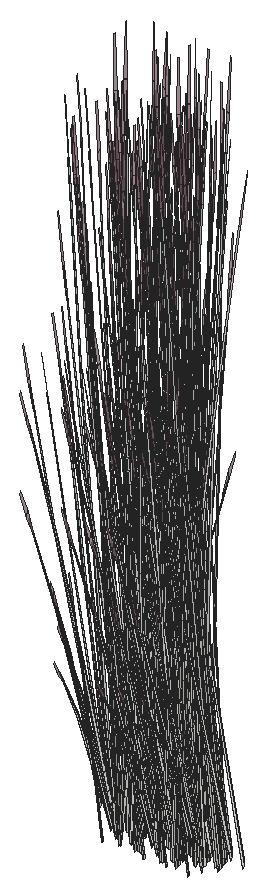
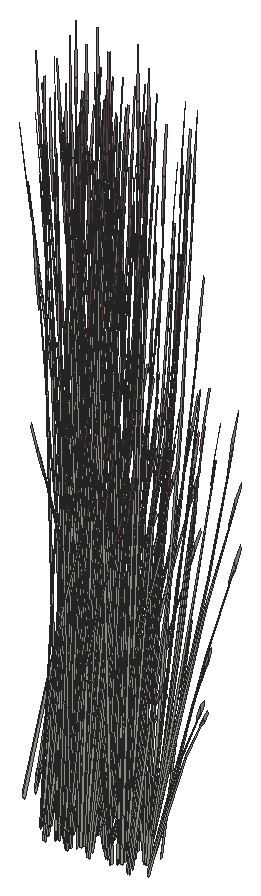
# SketchUp Ruby script. Lengths in inches.
U = 1.inch
M = Sketchup.active_model
def pt(a) = Geom::Point3d.new(a.map { |v| v * U })
def face(e, loops, mat)
  f = e.add_face(loops[0].map { |a| pt(a) })
  loops[1..].each { |l| e.add_face(l.map { |a| pt(a) }).erase! }
  f.material = f.back_material = mat if mat
  f
end
# faces: each face lists its corners as indices into pts; further lists are holes
def faces(e, pts, list, mat = nil) = list.each { |f| face(e, (f[0].is_a?(Array) ? f : [f]).map { |l| l.map { |i| pts[i] } }, mat) }
# xy, xz, yz: faces in a plane at the given z, y or x. An outline is a flat list of corners, or four numbers for a rectangle; further outlines are holes
def ring(l) = l.size == 4 ? [[l[0], l[1]], [l[2], l[1]], [l[2], l[3]], [l[0], l[3]]] : l.each_slice(2).to_a
def flat(e, list, mat, &to3) = list.each { |f| face(e, (f[0].is_a?(Array) ? f : [f]).map { |l| ring(l).map { |u, v| to3.(u, v) } }, mat) }
def xy(e, z, list, mat = nil) = flat(e, list, mat) { |x, y| [x, y, z] }
def xz(e, y, list, mat = nil) = flat(e, list, mat) { |x, z| [x, y, z] }
def yz(e, x, list, mat = nil) = flat(e, list, mat) { |y, z| [x, y, z] }
def lines(e, pts, list) = list.each { |a, b| e.add_line(pt(pts[a]), pt(pts[b])) }
# prism: a flat outline (further loops are holes) pulled along v
def prism(e, loops, v, mat = nil)
  f = face(e, loops, mat); d = Geom::Vector3d.new(v.map { |x| x * U })
  f.pushpull(f.normal.samedirection?(d) ? d.length : -d.length)
end
def box(e, o, s, mat = nil) = prism(e, [[o, [o[0] + s[0], o[1], o[2]], [o[0] + s[0], o[1] + s[1], o[2]], [o[0], o[1] + s[1], o[2]]]], [0, 0, s[2]], mat)
def at(x, y, z, deg = 0) = Geom::Transformation.translation(pt([x, y, z])) * Geom::Transformation.rotation(ORIGIN, Z_AXIS, deg.degrees)
def axes(o, x, y, z) = Geom::Transformation.new([*x, 0, *y, 0, *z, 0, *pt(o).to_a, 1])
def part(name) = M.definitions.add(name)
# library, detail: a bought-in or finely detailed component or shape, given as its bounding box
def library(name, o, s) = part(name).tap { |d| box(d.entities, o, s) }
def detail(e, o, s) = box(e.add_group.entities, o, s)
def put(e, d, t, mat = nil) = e.add_instance(d, t).tap { |i| i.material = mat if mat }
def group(e, t, mat = nil) = e.add_group.tap { |g| g.transformation = t; g.material = mat if mat }.entities
root = M.entities
M.materials.add("LightPink_Translucent").color = [144, 107, 117]
M.materials["LightPink_Translucent"].alpha = 0.75
c1 = part("blade")
p = [[2.15,0.21,22],[0,0.17,0],[0.09,0.45,0],[2.18,0.31,22],[2.29,0.31,22],[0.38,0.45,0],
  [2.48,0.24,33],[2.49,0.24,33],[2.48,0.22,33]]
faces(c1.entities,p,[[0,1,2,3],[4,5,2,3],[6,3,4,7],[8,0,3,6]])
c2 = part("seeds")
p = [[0.3,-0.1,1.38],[-0.01,-0.03,1.59],[-0.01,-0.03,0.03],[0.14,-0.07,-0.07],[0.29,-0.03,3],[0.15,0.01,3.11]]
faces(c2.entities,p,[[0,1,2,3],[1,0,4,5]],"LightPink_Translucent")
c3 = part("blade with seeds")
put(c3.entities,c1,at(0,0,0))
put(c3.entities,c2,axes([2.4,0.25,30.99],[1.5799,-0.05474,1.17369],[-0.12525,1.92788,0.29478],[-0.07173,-0.02425,1.56792]))
put(root,c3,axes([336.72,354.52,621.875],[0.14639,-0.01056,1.71376],[-0.09712,0.45778,0.13857],[-0.20862,-0.02831,0.73262]))
put(root,c3,axes([337.16,354.09,622.98],[-0.35281,-0.01123,-0.71045],[0.0237,-0.47284,0.08574],[-0.14947,-0.0499,1.00501]))
put(root,c3,axes([336.875,354.21,620.59],[0.06891,0.12984,1.43002],[-0.15879,0.35293,-0.30754],[-0.16304,-0.08436,0.61141]))
put(root,c3,axes([336.59,354.91,622.53],[-0.29332,-0.1301,-0.35414],[0.08555,-0.37955,0.4572],[-0.11809,0.0348,0.87481]))
put(root,c3,axes([337.04,354.1875,622.68],[-0.25628,0.30892,-0.51099],[-0.22444,-0.32634,-0.3958],[-0.13021,-0.047,0.97773]))
put(root,c3,axes([336.63,355.08,619.49],[0.00895,0.0735,1.76342],[-0.18044,0.38382,-0.26939],[-0.12817,-0.01935,0.30037]))
put(root,c3,axes([336.68,353.32,622.71],[0.02617,0.04654,1.77383],[-0.12614,0.41836,-0.16761],[-0.12775,0.00303,0.31391]))
put(root,c3,axes([336.66,354.86,622.73],[0.09971,-0.42522,0.48003],[0.32782,0.1454,0.3958],[-0.12892,0.02555,0.9933]))
put(root,c3,axes([337.18,353.87,623.03],[-0.0189,0.47427,-0.1216],[-0.35781,-0.01296,-0.67495],[-0.13781,-0.03295,1.02557]))
put(root,c3,axes([336.64,354.75,622.73],[-0.12963,-0.31798,0.0643],[0.23638,-0.15564,0.50621],[-0.1042,0.03071,0.77189]))
put(root,c3,axes([336.46,354.6,620.77],[0.22533,-0.03337,1.1486],[-0.14293,0.29403,0.84392],[-0.11135,-0.04411,0.25299]))
put(root,c3,axes([336.9,354.87,623.05],[0.29332,0.1301,0.35414],[-0.08555,0.37955,-0.4572],[-0.11809,0.0348,0.87481]))
put(root,c3,axes([337.81,355.75,620.06],[-0.36714,-0.07646,-0.62353],[0.07747,-0.47163,-0.16365],[-0.10956,-0.05715,1.37633]))
put(root,c3,axes([337.23,354.05,623.05],[0.20082,0.29199,0.35414],[-0.2293,0.2764,-0.4572],[-0.1165,-0.04206,0.87481]))
put(root,c3,axes([337.33,356.64,620.02],[-0.33032,-0.23318,-0.49651],[0.19744,-0.41812,0],[-0.07523,-0.05311,1.57504]))
put(root,c3,axes([336.97,353.4,620.13],[-0.10181,0.3808,-0.03893],[-0.31336,-0.11714,-0.17649],[-0.04758,-0.06228,0.58215]))
put(root,c3,axes([338.23,355.82,620.67],[-0.35635,0.30962,-0.29095],[-0.23697,-0.43749,-0.50002],[-0.08792,-0.04443,1.59708]))
put(root,c3,axes([336.8,355.14,620.375],[-0.44133,0,0],[0,-0.52122,-0.51607],[0,-0.11871,1.63711]))
put(root,c3,axes([337.42,356.46,620.03],[-0.08291,-0.40636,-0.30978],[0.32928,-0.11539,0.30978],[-0.06638,-0.04686,1.38974]))
put(root,c3,axes([337.14,355,620.33],[-0.32829,0.39208,0.30756],[-0.32849,-0.38796,-0.36492],[-0.01146,-0.11134,1.64885]))
put(root,c3,axes([338,355.6,620.21],[-0.21202,-0.39143,-0.44739],[0.32115,-0.27564,0.21531],[-0.06861,-0.04843,1.43643]))
put(root,c3,axes([340.4,354.44,621.875],[0.14639,-0.01056,1.71376],[-0.09712,0.45778,0.13857],[-0.20862,-0.02831,0.73262]))
put(root,c3,axes([338.03,355.82,620.4375],[0.09355,-0.55261,-0.23429],[0.44354,0.09633,0.51271],[-0.0775,-0.07631,1.5644]))
put(root,c3,axes([338.19,355.95,620.62],[-0.06809,0.4162,0.1448],[-0.33266,-0.07225,-0.41347],[-0.06054,-0.04274,1.26744]))
put(root,c3,axes([337.07,355.22,620.48],[0,0.46636,0.49651],[-0.39487,0,0],[0,-0.10622,1.57504]))
put(root,c3,axes([337.93,355.33,620.67],[-0.39748,-0.22252,-0.29095],[0.19139,-0.46966,-0.50002],[-0.01249,-0.11531,1.59708]))
put(root,c3,axes([341.16,354.77,621.34],[0.10032,-0.06746,1.77064],[0.0346,0.47103,0.13857],[-0.2173,0.0625,0.63284]))
put(root,c3,axes([337.07,354.8,620.03],[0.24637,-0.29097,-0.30978],[0.24637,0.29097,0.30978],[0,-0.09372,1.38974]))
put(root,c3,axes([338.08,355.55,620.36],[0.44609,0.09826,0.45755],[-0.09078,0.55493,0.17955],[-0.06519,-0.05359,1.58856]))
put(root,c3,axes([340.84,354.02,622.98],[-0.35281,-0.01123,-0.71045],[0.0237,-0.47284,0.08574],[-0.14947,-0.0499,1.00501]))
put(root,c3,axes([337.97,355.45,620.72],[-0.17124,0.42022,0.44739],[-0.35581,-0.20224,-0.21531],[0,-0.09687,1.43643]))
put(root,c3,axes([340.55,354.13,620.59],[0.06891,0.12984,1.43002],[-0.15879,0.35293,-0.30754],[-0.16304,-0.08436,0.61141]))
put(root,c3,axes([340.27,354.83,622.53],[-0.29332,-0.1301,-0.35414],[0.08555,-0.37955,0.4572],[-0.11809,0.0348,0.87481]))
put(root,c3,axes([337.84,356.44,620.47],[0.37926,-0.12378,0.17642],[0.09365,0.46065,0.35086],[-0.03382,-0.06712,1.60407]))
put(root,c3,axes([340.72,354.11,622.68],[-0.25628,0.30892,-0.51099],[-0.22444,-0.32634,-0.3958],[-0.13021,-0.047,0.97773]))
put(root,c3,axes([340.31,355,619.49],[0.00895,0.0735,1.76342],[-0.18044,0.38382,-0.26939],[-0.12817,-0.01935,0.30037]))
put(root,c3,axes([338.97,356.47,620.47],[0.10196,-0.46348,0.17642],[0.3731,0.13116,0.35086],[-0.06445,0.00226,1.60407]))
put(root,c3,axes([340.36,353.25,622.71],[0.02617,0.04654,1.77383],[-0.12614,0.41836,-0.16761],[-0.12775,0.00303,0.31391]))
put(root,c3,axes([338.71,355.5,620.3],[-0.32829,-0.4014,-0.06131],[0.32849,-0.40164,0],[-0.01146,-0.01402,1.75571]))
put(root,c3,axes([340.34,354.79,622.73],[0.09971,-0.42522,0.48003],[0.32782,0.1454,0.3958],[-0.12892,0.02555,0.9933]))
put(root,c3,axes([340.85,353.79,623.03],[-0.0189,0.47427,-0.1216],[-0.35781,-0.01296,-0.67495],[-0.13781,-0.03295,1.02557]))
put(root,c3,axes([338.04,355.04,620.36],[0.15345,0.52148,0.45755],[-0.43845,0.18134,0.17955],[0.00536,-0.09582,1.58856]))
put(root,c3,axes([340.3125,354.67,622.73],[-0.12963,-0.31798,0.0643],[0.23638,-0.15564,0.50621],[-0.1042,0.03071,0.77189]))
put(root,c3,axes([338.41,356.33,620.2],[-0.11516,-0.40207,0],[0.32884,-0.1408,0],[0,0,1.54371]))
put(root,c3,axes([340.14,354.52,620.77],[0.22533,-0.03337,1.1486],[-0.14293,0.29403,0.84392],[-0.11135,-0.04411,0.25299]))
put(root,c3,axes([342.27,354.54,621.875],[0.14639,-0.01056,1.71376],[-0.09712,0.45778,0.13857],[-0.20862,-0.02831,0.73262]))
put(root,c3,axes([338.6,355.09,620.21],[0,-0.53961,0],[0.44133,0,0],[0,0,1.79456]))
put(root,c3,axes([338.18,355.19,620.43],[0.39767,0.22603,0.24065],[-0.19139,0.46966,0.50002],[0,-0.10827,1.60543]))
put(root,c3,axes([338.06,354.87,620.72],[-0.38326,0.02879,0.44739],[-0.03466,-0.47788,-0.21531],[0.06861,-0.04843,1.43643]))
put(root,c3,axes([337.88,354.05,620.47],[-0.10196,0.46348,0.17642],[-0.3731,-0.13116,0.35086],[0.06445,-0.00226,1.60407]))
put(root,c3,axes([340.58,354.79,623.05],[0.29332,0.1301,0.35414],[-0.08555,0.37955,-0.4572],[-0.11809,0.0348,0.87481]))
put(root,c3,axes([341.49,355.67,620.06],[-0.36714,-0.07646,-0.62353],[0.07747,-0.47163,-0.16365],[-0.10956,-0.05715,1.37633]))
put(root,c3,axes([340.91,353.97,623.05],[0.20082,0.29199,0.35414],[-0.2293,0.2764,-0.4572],[-0.1165,-0.04206,0.87481]))
put(root,c3,axes([339.01,354.08,620.47],[-0.37926,0.12378,0.17642],[-0.09365,-0.46065,0.35086],[0.03382,0.06712,1.60407]))
put(root,c3,axes([338.39,354.75,620.36],[-0.29264,0.42323,0.45755],[-0.34767,-0.3736,0.17955],[0.07055,-0.04224,1.58856]))
put(root,c3,axes([338.89,355.41,620.21],[0.24637,0.30123,0],[-0.24637,0.30123,0],[0,0,1.69266]))
put(root,c3,axes([341.01,356.56,620.02],[-0.33032,-0.23318,-0.49651],[0.19744,-0.41812,0],[-0.07523,-0.05311,1.57504]))
put(root,c3,axes([338.77,354.96,620.38],[-0.44609,-0.09826,0.49198],[0.09078,-0.55493,0.19306],[0.06519,0.05359,1.70813]))
put(root,c3,axes([338.89,355.21,620.21],[0.39487,0,0],[0,0.48281,0],[0,0,1.78407]))
put(root,c3,axes([342.71,354.12,622.98],[-0.35281,-0.01123,-0.71045],[0.0237,-0.47284,0.08574],[-0.14947,-0.0499,1.00501]))
put(root,c3,axes([338.51,354.67,620.72],[-0.21202,-0.39143,0.44739],[0.32115,-0.27564,-0.21531],[0.06861,0.04843,1.43643]))
put(root,c3,axes([338.13,354.77,620.67],[-0.04113,-0.53214,-0.29095],[0.42835,-0.03218,-0.50002],[0.07543,-0.07088,1.59708]))
put(root,c3,axes([342.42,354.23,620.59],[0.06891,0.12984,1.43002],[-0.15879,0.35293,-0.30754],[-0.16304,-0.08436,0.61141]))
put(root,c3,axes([340.65,353.32,620.13],[-0.10181,0.3808,-0.03893],[-0.31336,-0.11714,-0.17649],[-0.04758,-0.06228,0.58215]))
put(root,c3,axes([342.14,354.93,622.53],[-0.29332,-0.1301,-0.35414],[0.08555,-0.37955,0.4572],[-0.11809,0.0348,0.87481]))
put(root,c3,axes([338.07,353.59,620.03],[0.32928,0.11539,-0.30978],[-0.08291,0.40636,0.30978],[0.06638,-0.04686,1.38974]))
put(root,c3,axes([341.9,355.74,620.67],[-0.35635,0.30962,-0.29095],[-0.23697,-0.43749,-0.50002],[-0.08792,-0.04443,1.59708]))
put(root,c3,axes([342.59,354.21,622.68],[-0.25628,0.30892,-0.51099],[-0.22444,-0.32634,-0.3958],[-0.13021,-0.047,0.97773]))
put(root,c3,axes([342.18,355.1,619.49],[0.00895,0.0735,1.76342],[-0.18044,0.38382,-0.26939],[-0.12817,-0.01935,0.30037]))
put(root,c3,axes([340.48,355.0625,620.375],[-0.44133,0,0],[0,-0.52122,-0.51607],[0,-0.11871,1.63711]))
put(root,c3,axes([341.1,356.39,620.03],[-0.08291,-0.40636,-0.30978],[0.32928,-0.11539,0.30978],[-0.06638,-0.04686,1.38974]))
put(root,c3,axes([338.66,354.57,620.62],[0.06809,-0.4162,0.1448],[0.33266,0.07225,-0.41347],[0.06054,0.04274,1.26744]))
put(root,c3,axes([342.23,353.35,622.71],[0.02617,0.04654,1.77383],[-0.12614,0.41836,-0.16761],[-0.12775,0.00303,0.31391]))
put(root,c3,axes([339.13,353.84,620.48],[-0.33032,-0.23318,0.49651],[0.19744,-0.41812,0],[0.07523,0.05311,1.57504]))
put(root,c3,axes([340.82,354.92,620.33],[-0.32829,0.39208,0.30756],[-0.32849,-0.38796,-0.36492],[-0.01146,-0.11134,1.64885]))
put(root,c3,axes([342.21,354.89,622.73],[0.09971,-0.42522,0.48003],[0.32782,0.1454,0.3958],[-0.12892,0.02555,0.9933]))
put(root,c3,axes([342.73,353.89,623.03],[-0.0189,0.47427,-0.1216],[-0.35781,-0.01296,-0.67495],[-0.13781,-0.03295,1.02557]))
put(root,c3,axes([338.84,356.28,620.18],[0.37054,-0.15823,-0.19198],[0.1302,0.45581,0.00008],[0.0409,-0.01749,1.73897]))
put(root,c3,axes([342.5,353.92,622.53],[-0.20082,-0.29199,-0.35414],[0.2293,-0.2764,0.4572],[-0.1165,-0.04206,0.87481]))
put(root,c3,axes([342.18,354.77,622.73],[-0.12963,-0.31798,0.0643],[0.23638,-0.15564,0.50621],[-0.1042,0.03071,0.77189]))
put(root,c3,axes([341.68,355.52,620.21],[-0.21202,-0.39143,-0.44739],[0.32115,-0.27564,0.21531],[-0.06861,-0.04843,1.43643]))
put(root,c3,axes([342.01,354.62,620.77],[0.22533,-0.03337,1.1486],[-0.14293,0.29403,0.84392],[-0.11135,-0.04411,0.25299]))
put(root,c3,axes([341.71,355.74,620.4375],[0.09355,-0.55261,-0.23429],[0.44354,0.09633,0.51271],[-0.0775,-0.07631,1.5644]))
put(root,c3,axes([341.87,355.87,620.62],[-0.06809,0.4162,0.1448],[-0.33266,-0.07225,-0.41347],[-0.06054,-0.04274,1.26744]))
put(root,c3,axes([340.75,355.14,620.48],[0,0.46636,0.49651],[-0.39487,0,0],[0,-0.10622,1.57504]))
put(root,c3,axes([339.43,354.05,620.03],[0.08291,0.40636,-0.30978],[-0.32928,0.11539,0.30978],[0.06638,0.04686,1.38974]))
put(root,c3,axes([342.45,354.89,623.05],[0.29332,0.1301,0.35414],[-0.08555,0.37955,-0.4572],[-0.11809,0.0348,0.87481]))
put(root,c3,axes([344.32,354.45,621.875],[0.14639,-0.01056,1.71376],[-0.09712,0.45778,0.13857],[-0.20862,-0.02831,0.73262]))
put(root,c3,axes([338.625,354.7,620.67],[0.35635,-0.30962,-0.29095],[0.23697,0.43749,-0.50002],[0.08792,0.04443,1.59708]))
put(root,c3,axes([339.68,354.65,623.05],[-0.30722,0.06665,0.35414],[-0.08112,-0.381,-0.4572],[0.08804,-0.10234,0.87481]))
put(root,c3,axes([341.61,355.25,620.67],[-0.39748,-0.22252,-0.29095],[0.19139,-0.46966,-0.50002],[-0.01249,-0.11531,1.59708]))
put(root,c3,axes([343.36,355.77,620.06],[-0.36714,-0.07646,-0.62353],[0.07747,-0.47163,-0.16365],[-0.10956,-0.05715,1.37633]))
put(root,c3,axes([342.78,354.07,623.05],[0.20082,0.29199,0.35414],[-0.2293,0.2764,-0.4572],[-0.1165,-0.04206,0.87481]))
put(root,c3,axes([337.72,354.42,619.59],[-0.3474,0.18671,1.28929],[-0.11057,-0.53572,0.50096],[0.21332,0.00891,1.46642]))
put(root,c3,axes([342.875,356.66,620.02],[-0.33032,-0.23318,-0.49651],[0.19744,-0.41812,0],[-0.07523,-0.05311,1.57504]))
put(root,c3,axes([340.75,354.72,620.03],[0.24637,-0.29097,-0.30978],[0.24637,0.29097,0.30978],[0,-0.09372,1.38974]))
put(root,c3,axes([341.76,355.48,620.36],[0.44609,0.09826,0.45755],[-0.09078,0.55493,0.17955],[-0.06519,-0.05359,1.58856]))
put(root,c3,axes([339.32,353.6,620.375],[0.22066,-0.46731,0],[0.36918,0.26061,-0.51607],[0.08408,0.05936,1.63711]))
put(root,c3,axes([345.08,354.78,621.34],[0.10032,-0.06746,1.77064],[0.0346,0.47103,0.13857],[-0.2173,0.0625,0.63284]))
put(root,c3,axes([339.52,353.88,620.02],[0.33032,0.23318,-0.49651],[-0.19744,0.41812,0],[0.07523,0.05311,1.57504]))
put(root,c3,axes([341.64,355.375,620.72],[-0.17124,0.42022,0.44739],[-0.35581,-0.20224,-0.21531],[0,-0.09687,1.43643]))
put(root,c3,axes([342.52,353.42,620.13],[-0.10181,0.3808,-0.03893],[-0.31336,-0.11714,-0.17649],[-0.04758,-0.06228,0.58215]))
put(root,c3,axes([339.73,355.56,623.05],[-0.29332,-0.1301,0.35414],[0.08555,-0.37955,-0.4572],[0.11809,-0.0348,0.87481]))
put(root,c3,axes([341.52,356.36,620.47],[0.37926,-0.12378,0.17642],[0.09365,0.46065,0.35086],[-0.03382,-0.06712,1.60407]))
put(root,c3,axes([344.75,354.03,622.98],[-0.35281,-0.01123,-0.71045],[0.0237,-0.47284,0.08574],[-0.14947,-0.0499,1.00501]))
put(root,c3,axes([340.6,355.05,620.26],[-0.21881,-0.29821,-0.06488],[0.23965,-0.27324,-0.29416],[0.0679,-0.01924,0.97024]))
put(root,c3,axes([344.47,354.14,620.59],[0.06891,0.12984,1.43002],[-0.15879,0.35293,-0.30754],[-0.16304,-0.08436,0.61141]))
put(root,c3,axes([343.78,355.84,620.67],[-0.35635,0.30962,-0.29095],[-0.23697,-0.43749,-0.50002],[-0.08792,-0.04443,1.59708]))
put(root,c3,axes([344.1875,354.84,622.53],[-0.29332,-0.1301,-0.35414],[0.08555,-0.37955,0.4572],[-0.11809,0.0348,0.87481]))
put(root,c3,axes([339.96,354.59,622.73],[0.2423,0.19613,0.0643],[-0.14107,0.2793,0.50621],[0.07768,-0.0903,0.77189]))
put(root,c3,axes([342.65,356.39,620.47],[0.10196,-0.46348,0.17642],[0.3731,0.13116,0.35086],[-0.06445,0.00226,1.60407]))
put(root,c3,axes([342.35,355.16,620.375],[-0.44133,0,0],[0,-0.52122,-0.51607],[0,-0.11871,1.63711]))
put(root,c3,axes([342.97,356.49,620.03],[-0.08291,-0.40636,-0.30978],[0.32928,-0.11539,0.30978],[-0.06638,-0.04686,1.38974]))
put(root,c3,axes([342.38,355.43,620.3],[-0.32829,-0.4014,-0.06131],[0.32849,-0.40164,0],[-0.01146,-0.01402,1.75571]))
put(root,c3,axes([339.89,354.5,622.73],[0.08753,0.42921,0.48003],[-0.34336,0.07449,0.3958],[0.1012,-0.10094,0.9933]))
put(root,c3,axes([344.64,354.12,622.68],[-0.25628,0.30892,-0.51099],[-0.22444,-0.32634,-0.3958],[-0.13021,-0.047,0.97773]))
put(root,c3,axes([344.22,355.01,619.49],[0.00895,0.0735,1.76342],[-0.18044,0.38382,-0.26939],[-0.12817,-0.01935,0.30037]))
put(root,c3,axes([342.69,355.03,620.33],[-0.32829,0.39208,0.30756],[-0.32849,-0.38796,-0.36492],[-0.01146,-0.11134,1.64885]))
put(root,c3,axes([341.72,354.97,620.36],[0.15345,0.52148,0.45755],[-0.43845,0.18134,0.17955],[0.00536,-0.09582,1.58856]))
put(root,c3,axes([344.27,353.26,622.71],[0.02617,0.04654,1.77383],[-0.12614,0.41836,-0.16761],[-0.12775,0.00303,0.31391]))
put(root,c3,axes([342.09,356.25,620.2],[-0.11516,-0.40207,0],[0.32884,-0.1408,0],[0,0,1.54371]))
put(root,c3,axes([340,355.68,622.73],[0.12963,0.31798,0.0643],[-0.23638,0.15564,0.50621],[0.1042,-0.03071,0.77189]))
put(root,c3,axes([343.55,355.62,620.21],[-0.21202,-0.39143,-0.44739],[0.32115,-0.27564,0.21531],[-0.06861,-0.04843,1.43643]))
put(root,c3,axes([339.85,355.6875,623.03],[-0.17758,-0.42229,-0.1216],[0.31518,-0.20752,-0.67495],[0.13282,-0.05572,1.02557]))
put(root,c3,axes([339.97,355.5625,622.73],[-0.09971,0.42522,0.48003],[-0.32782,-0.1454,0.3958],[0.12892,-0.02555,0.9933]))
put(root,c3,axes([344.25,354.8,622.73],[0.09971,-0.42522,0.48003],[0.32782,0.1454,0.3958],[-0.12892,0.02555,0.9933]))
put(root,c3,axes([344.77,353.8,623.03],[-0.0189,0.47427,-0.1216],[-0.35781,-0.01296,-0.67495],[-0.13781,-0.03295,1.02557]))
put(root,c3,axes([344.23,354.68,622.73],[-0.12963,-0.31798,0.0643],[0.23638,-0.15564,0.50621],[-0.1042,0.03071,0.77189]))
put(root,c3,axes([343.23,355.21,620.47],[-0.2773,-0.3397,0.17642],[0.27945,-0.32949,0.35086],[-0.03063,0.06937,1.60407]))
put(root,c3,axes([344.06,354.53,620.77],[0.22533,-0.03337,1.1486],[-0.14293,0.29403,0.84392],[-0.11135,-0.04411,0.25299]))
put(root,c3,axes([342.27,355.01,620.21],[0,-0.53961,0],[0.44133,0,0],[0,0,1.79456]))
put(root,c3,axes([341.86,355.11,620.43],[0.39767,0.22603,0.24065],[-0.19139,0.46966,0.50002],[0,-0.10827,1.60543]))
put(root,c3,axes([343.58,355.84,620.4375],[0.09355,-0.55261,-0.23429],[0.44354,0.09633,0.51271],[-0.0775,-0.07631,1.5644]))
put(root,c3,axes([341.73,354.79,620.72],[-0.38326,0.02879,0.44739],[-0.03466,-0.47788,-0.21531],[0.06861,-0.04843,1.43643]))
put(root,c3,axes([339.84,355.32,622.68],[0.09562,-0.42421,-0.51099],[0.32782,0.1454,-0.3958],[0.13199,-0.0389,0.97773]))
put(root,c3,axes([343.74,355.97,620.62],[-0.06809,0.4162,0.1448],[-0.33266,-0.07225,-0.41347],[-0.06054,-0.04274,1.26744]))
put(root,c3,axes([341.56,353.97,620.47],[-0.10196,0.46348,0.17642],[-0.3731,-0.13116,0.35086],[0.06445,-0.00226,1.60407]))
put(root,c3,axes([342.62,355.24,620.48],[0,0.46636,0.49651],[-0.39487,0,0],[0,-0.10622,1.57504]))
put(root,c3,axes([340.04,355.52,622.53],[0.29332,0.1301,-0.35414],[-0.08555,0.37955,0.4572],[0.11809,-0.0348,0.87481]))
put(root,c3,axes([343.48,355.35,620.67],[-0.39748,-0.22252,-0.29095],[0.19139,-0.46966,-0.50002],[-0.01249,-0.11531,1.59708]))
put(root,c3,axes([342.68,354,620.47],[-0.37926,0.12378,0.17642],[-0.09365,-0.46065,0.35086],[0.03382,0.06712,1.60407]))
put(root,c3,axes([340.1875,355.44,619.98],[-0.22732,0.05597,1.41583],[-0.03618,-0.44548,0.08104],[0.15921,-0.06743,0.80566]))
put(root,c3,axes([344.5,354.8,623.05],[0.29332,0.1301,0.35414],[-0.08555,0.37955,-0.4572],[-0.11809,0.0348,0.87481]))
put(root,c3,axes([340.4375,355.15,619.49],[-0.01845,-0.0708,1.76342],[0.12793,-0.41416,-0.26939],[0.12905,-0.00596,0.30037]))
put(root,c3,axes([339.24,355.05,621.875],[-0.14639,0.01056,1.71376],[0.09712,-0.45778,0.13857],[0.20862,0.02831,0.73262]))
put(root,c3,axes([342.0625,354.67,620.36],[-0.29264,0.42323,0.45755],[-0.34767,-0.3736,0.17955],[0.07055,-0.04224,1.58856]))
put(root,c3,axes([342.5625,355.34,620.21],[0.24637,0.30123,0],[-0.24637,0.30123,0],[0,0,1.69266]))
put(root,c3,axes([345.4,355.68,620.06],[-0.36714,-0.07646,-0.62353],[0.07747,-0.47163,-0.16365],[-0.10956,-0.05715,1.37633]))
put(root,c3,axes([344.83,353.98,623.05],[0.20082,0.29199,0.35414],[-0.2293,0.2764,-0.4572],[-0.1165,-0.04206,0.87481]))
put(root,c3,axes([339.78,355.48,622.98],[0.31014,-0.20596,-0.71045],[0.17284,0.42397,0.08574],[0.14985,-0.04816,1.00501]))
put(root,c3,axes([342.45,354.88,620.38],[-0.44609,-0.09826,0.49198],[0.09078,-0.55493,0.19306],[0.06519,0.05359,1.70813]))
put(root,c3,axes([342.62,354.82,620.03],[0.24637,-0.29097,-0.30978],[0.24637,0.29097,0.30978],[0,-0.09372,1.38974]))
put(root,c3,axes([343.63,355.58,620.36],[0.44609,0.09826,0.45755],[-0.09078,0.55493,0.17955],[-0.06519,-0.05359,1.58856]))
put(root,c3,axes([340.82,355.02,622.72],[0.04898,-0.07104,1.74944],[-0.06269,-0.43574,-0.27667],[0.12289,-0.08262,0.14031]))
put(root,c3,axes([344.92,356.57,620.02],[-0.33032,-0.23318,-0.49651],[0.19744,-0.41812,0],[-0.07523,-0.05311,1.57504]))
put(root,c3,axes([342.57,355.13,620.21],[0.39487,0,0],[0,0.48281,0],[0,0,1.78407]))
put(root,c3,axes([343.52,355.48,620.72],[-0.17124,0.42022,0.44739],[-0.35581,-0.20224,-0.21531],[0,-0.09687,1.43643]))
put(root,c3,axes([342.19,354.6,620.72],[-0.21202,-0.39143,0.44739],[0.32115,-0.27564,-0.21531],[0.06861,0.04843,1.43643]))
put(root,c3,axes([343.39,356.46,620.47],[0.37926,-0.12378,0.17642],[0.09365,0.46065,0.35086],[-0.03382,-0.06712,1.60407]))
put(root,c3,axes([341.75,353.51,620.03],[0.32928,0.11539,-0.30978],[-0.08291,0.40636,0.30978],[0.06638,-0.04686,1.38974]))
put(root,c3,axes([344.5625,353.33,620.13],[-0.10181,0.3808,-0.03893],[-0.31336,-0.11714,-0.17649],[-0.04758,-0.06228,0.58215]))
put(root,c3,axes([344.52,356.49,620.47],[0.10196,-0.46348,0.17642],[0.3731,0.13116,0.35086],[-0.06445,0.00226,1.60407]))
put(root,c3,axes([342.34,354.49,620.62],[0.06809,-0.4162,0.1448],[0.33266,0.07225,-0.41347],[0.06054,0.04274,1.26744]))
put(root,c3,axes([344.26,355.53,620.3],[-0.32829,-0.4014,-0.06131],[0.32849,-0.40164,0],[-0.01146,-0.01402,1.75571]))
put(root,c3,axes([345.82,355.75,620.67],[-0.35635,0.30962,-0.29095],[-0.23697,-0.43749,-0.50002],[-0.08792,-0.04443,1.59708]))
put(root,c3,axes([342.81,353.76,620.48],[-0.33032,-0.23318,0.49651],[0.19744,-0.41812,0],[0.07523,0.05311,1.57504]))
put(root,c3,axes([344.39,355.07,620.375],[-0.44133,0,0],[0,-0.52122,-0.51607],[0,-0.11871,1.63711]))
put(root,c3,axes([345.01,356.4,620.03],[-0.08291,-0.40636,-0.30978],[0.32928,-0.11539,0.30978],[-0.06638,-0.04686,1.38974]))
put(root,c3,axes([347.38,354.2,621.875],[0.14639,-0.01056,1.71376],[-0.09712,0.45778,0.13857],[-0.20862,-0.02831,0.73262]))
put(root,c3,axes([343.59,355.07,620.36],[0.15345,0.52148,0.45755],[-0.43845,0.18134,0.17955],[0.00536,-0.09582,1.58856]))
put(root,c3,axes([342.52,356.2,620.18],[0.37054,-0.15823,-0.19198],[0.1302,0.45581,0.00008],[0.0409,-0.01749,1.73897]))
put(root,c3,axes([343.52,355,620.21],[0.17124,-0.42022,-0.44739],[0.35581,0.20224,0.21531],[0,-0.09687,1.43643]))
put(root,c3,axes([343.96,356.35,620.2],[-0.11516,-0.40207,0],[0.32884,-0.1408,0],[0,0,1.54371]))
put(root,c3,axes([344.74,354.93,620.33],[-0.32829,0.39208,0.30756],[-0.32849,-0.38796,-0.36492],[-0.01146,-0.11134,1.64885]))
put(root,c3,axes([345.59,355.53,620.21],[-0.21202,-0.39143,-0.44739],[0.32115,-0.27564,0.21531],[-0.06861,-0.04843,1.43643]))
put(root,c3,axes([344.14,355.11,620.21],[0,-0.53961,0],[0.44133,0,0],[0,0,1.79456]))
put(root,c3,axes([343.73,355.21,620.43],[0.39767,0.22603,0.24065],[-0.19139,0.46966,0.50002],[0,-0.10827,1.60543]))
put(root,c3,axes([343.61,354.89,620.72],[-0.38326,0.02879,0.44739],[-0.03466,-0.47788,-0.21531],[0.06861,-0.04843,1.43643]))
put(root,c3,axes([343.11,353.97,620.03],[0.08291,0.40636,-0.30978],[-0.32928,0.11539,0.30978],[0.06638,0.04686,1.38974]))
put(root,c3,axes([348.14,354.53,621.34],[0.10032,-0.06746,1.77064],[0.0346,0.47103,0.13857],[-0.2173,0.0625,0.63284]))
put(root,c3,axes([343.43,354.07,620.47],[-0.10196,0.46348,0.17642],[-0.3731,-0.13116,0.35086],[0.06445,-0.00226,1.60407]))
put(root,c3,axes([345.625,355.75,620.4375],[0.09355,-0.55261,-0.23429],[0.44354,0.09633,0.51271],[-0.0775,-0.07631,1.5644]))
put(root,c3,axes([342.3,354.62,620.67],[0.35635,-0.30962,-0.29095],[0.23697,0.43749,-0.50002],[0.08792,0.04443,1.59708]))
put(root,c3,axes([343.36,354.57,623.05],[-0.30722,0.06665,0.35414],[-0.08112,-0.381,-0.4572],[0.08804,-0.10234,0.87481]))
put(root,c3,axes([345.79,355.88,620.62],[-0.06809,0.4162,0.1448],[-0.33266,-0.07225,-0.41347],[-0.06054,-0.04274,1.26744]))
put(root,c3,axes([344.66,355.15,620.48],[0,0.46636,0.49651],[-0.39487,0,0],[0,-0.10622,1.57504]))
put(root,c3,axes([344.56,354.1,620.47],[-0.37926,0.12378,0.17642],[-0.09365,-0.46065,0.35086],[0.03382,0.06712,1.60407]))
put(root,c3,axes([347.82,353.78,622.98],[-0.35281,-0.01123,-0.71045],[0.0237,-0.47284,0.08574],[-0.14947,-0.0499,1.00501]))
put(root,c3,axes([347.25,354.59,622.53],[-0.29332,-0.1301,-0.35414],[0.08555,-0.37955,0.4572],[-0.11809,0.0348,0.87481]))
put(root,c3,axes([343.9375,354.77,620.36],[-0.29264,0.42323,0.45755],[-0.34767,-0.3736,0.17955],[0.07055,-0.04224,1.58856]))
put(root,c3,axes([344.4375,355.4375,620.21],[0.24637,0.30123,0],[-0.24637,0.30123,0],[0,0,1.69266]))
put(root,c3,axes([341.4,354.35,619.59],[-0.3474,0.18671,1.28929],[-0.11057,-0.53572,0.50096],[0.21332,0.00891,1.46642]))
put(root,c3,axes([345.52,355.26,620.67],[-0.39748,-0.22252,-0.29095],[0.19139,-0.46966,-0.50002],[-0.01249,-0.11531,1.59708]))
put(root,c3,axes([344.32,354.98,620.38],[-0.44609,-0.09826,0.49198],[0.09078,-0.55493,0.19306],[0.06519,0.05359,1.70813]))
put(root,c3,axes([343,353.52,620.375],[0.22066,-0.46731,0],[0.36918,0.26061,-0.51607],[0.08408,0.05936,1.63711]))
